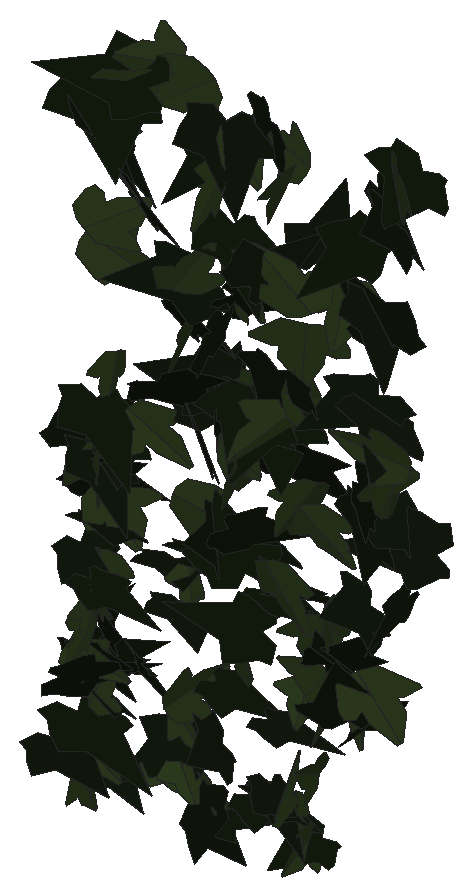
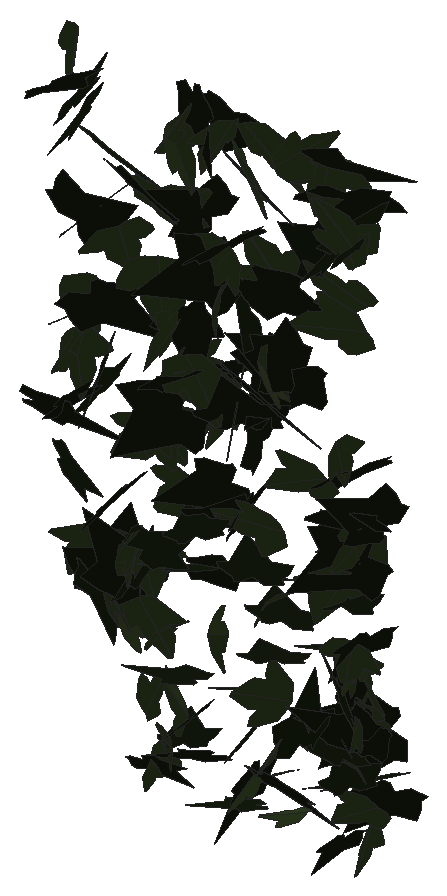
# SketchUp Ruby script. Lengths in inches.
U = 1.inch
M = Sketchup.active_model
def pt(a) = Geom::Point3d.new(a.map { |v| v * U })
def face(e, loops, mat)
  f = e.add_face(loops[0].map { |a| pt(a) })
  loops[1..].each { |l| e.add_face(l.map { |a| pt(a) }).erase! }
  f.material = f.back_material = mat if mat
  f
end
# faces: each face lists its corners as indices into pts; further lists are holes
def faces(e, pts, list, mat = nil) = list.each { |f| face(e, (f[0].is_a?(Array) ? f : [f]).map { |l| l.map { |i| pts[i] } }, mat) }
# xy, xz, yz: faces in a plane at the given z, y or x. An outline is a flat list of corners, or four numbers for a rectangle; further outlines are holes
def ring(l) = l.size == 4 ? [[l[0], l[1]], [l[2], l[1]], [l[2], l[3]], [l[0], l[3]]] : l.each_slice(2).to_a
def flat(e, list, mat, &to3) = list.each { |f| face(e, (f[0].is_a?(Array) ? f : [f]).map { |l| ring(l).map { |u, v| to3.(u, v) } }, mat) }
def xy(e, z, list, mat = nil) = flat(e, list, mat) { |x, y| [x, y, z] }
def xz(e, y, list, mat = nil) = flat(e, list, mat) { |x, z| [x, y, z] }
def yz(e, x, list, mat = nil) = flat(e, list, mat) { |y, z| [x, y, z] }
def lines(e, pts, list) = list.each { |a, b| e.add_line(pt(pts[a]), pt(pts[b])) }
# prism: a flat outline (further loops are holes) pulled along v
def prism(e, loops, v, mat = nil)
  f = face(e, loops, mat); d = Geom::Vector3d.new(v.map { |x| x * U })
  f.pushpull(f.normal.samedirection?(d) ? d.length : -d.length)
end
def box(e, o, s, mat = nil) = prism(e, [[o, [o[0] + s[0], o[1], o[2]], [o[0] + s[0], o[1] + s[1], o[2]], [o[0], o[1] + s[1], o[2]]]], [0, 0, s[2]], mat)
def at(x, y, z, deg = 0) = Geom::Transformation.translation(pt([x, y, z])) * Geom::Transformation.rotation(ORIGIN, Z_AXIS, deg.degrees)
def axes(o, x, y, z) = Geom::Transformation.new([*x, 0, *y, 0, *z, 0, *pt(o).to_a, 1])
def part(name) = M.definitions.add(name)
# library, detail: a bought-in or finely detailed component or shape, given as its bounding box
def library(name, o, s) = part(name).tap { |d| box(d.entities, o, s) }
def detail(e, o, s) = box(e.add_group.entities, o, s)
def put(e, d, t, mat = nil) = e.add_instance(d, t).tap { |i| i.material = mat if mat }
def group(e, t, mat = nil) = e.add_group.tap { |g| g.transformation = t; g.material = mat if mat }.entities
root = M.entities
M.materials.add("1026 AP 7946 SUNNY SIDE UP").color = [254, 231, 186]
M.materials.add("efeu1").color = [18, 25, 13]
M.materials.add("efeu2").color = [43, 57, 29]
c1 = part("ivyleaf_9")
p = [[1.54,2.16,1.25],[1.36,2.04,1.19],[-0.21,0.99,0.68],[-0.71,1.11,0.82],[-0.85,0.86,0.67],[-0.8,0.17,0.21],
  [-0.9,-0.01,0.1],[-0.67,-0.16,-0.02],[-0.08,-0.08,-0.05],[-0.03,-0.6,-0.4],[0.65,-0.88,-0.66],[0.83,-0.6,-0.49],
  [1.29,-0.42,-0.43],[1.8125,-0.07,-0.26],[1.21,0.44,0.15]]
faces(c1.entities,p,[[0,1,2,3,4,5,6,7,8,9,10,11,12,13,14]],"efeu1")
c2 = part("ivyleaf_10")
p = [[0,0.5,-0.03],[-0.0625,2.02,-0.43],[-0.19,2.01,-0.46],[-0.54,1.05,-0.29],[-0.52,0.625,-0.18],[-0.83,0.76,-0.28],
  [-1.16,0.64,-0.33],[-1.15,0.33,-0.24],[-0.77,-0.39,0.02],[-0.3,-0.51,0.16],[0.04,-0.48,0.23],[-0.02,2.01,-0.4375],
  [-0.06,2.01,-0.43],[0.04,-0.49,0.23],[0.67,-0.49,0.14],[1.38,0.36,-0.2],[1.375,0.51,-0.24],[0.81,0.65,-0.19],
  [0.62,0.59,-0.15],[0.6,1.09,-0.28],[0.5,1.23,-0.31]]
faces(c2.entities,p,[[0,1,2,3,4,5,6,7,8,9,10],[11,12,0,13,14,15,16,17,18,19,20]],"efeu2")
put(root,c1,axes([140.07,210.01,274.99],[0.40178,0.27327,0.06244],[0.08476,0.03035,-0.38477],[-0.43136,0.26049,-0.01745]),"1026 AP 7946 SUNNY SIDE UP")
put(root,c1,axes([138.16,210.15,268.72],[-0.04545,-0.15248,-0.27536],[0.07021,0.26267,-0.15833],[0.47756,-0.05313,-0.00293]),"1026 AP 7946 SUNNY SIDE UP")
put(root,c2,axes([140.75,210.3125,278.22],[0.38972,-0.31524,0.01139],[-0.01605,-0.02434,-0.41257],[0.49583,0.24698,-0.0223]),"1026 AP 7946 SUNNY SIDE UP")
put(root,c2,axes([142.29,210.24,276.97],[0.41137,0.1162,0.24439],[-0.36093,-0.06335,0.2932],[0.20366,-0.34698,0.02599]),"1026 AP 7946 SUNNY SIDE UP")
put(root,c1,axes([143.24,210.53,273.7],[-0.01,-0.29094,0.24842],[-0.01209,-0.24268,-0.30121],[0.59572,-0.00981,-0.00194]),"1026 AP 7946 SUNNY SIDE UP")
put(root,c2,axes([141.83,210.3,272.5],[-0.43233,0.13643,-0.20668],[0.24343,-0.13631,-0.31365],[-0.29504,-0.31238,0.04407]),"1026 AP 7946 SUNNY SIDE UP")
put(root,c2,axes([140.28,210.22,276.53],[-0.24834,-0.27881,0.12117],[0.07338,0.11045,0.33049],[-0.47111,0.16418,-0.01239]),"1026 AP 7946 SUNNY SIDE UP")
put(root,c2,axes([141.3125,210.05,274.09],[0.037,-0.24145,-0.32858],[0.04753,0.31829,-0.24513],[0.62549,-0.0099,0.03806]),"1026 AP 7946 SUNNY SIDE UP")
put(root,c2,axes([141.61,210.55,274.69],[-0.09782,-0.18167,0.35137],[-0.02071,-0.34529,-0.19339],[0.60871,-0.04095,0.04988]),"1026 AP 7946 SUNNY SIDE UP")
put(root,c2,axes([138.46,210.39,270.53],[0.3277,-0.2593,0.03455],[0.00983,-0.03981,-0.34233],[0.4113,0.20754,-0.01935]),"1026 AP 7946 SUNNY SIDE UP")
put(root,c1,axes([140.87,210.43,279.06],[-0.41385,-0.1169,-0.29365],[0.4378,0.06819,-0.29395],[0.20511,-0.38143,0.03493]),"1026 AP 7946 SUNNY SIDE UP")
put(root,c2,axes([143.83,210.3,274.96],[-0.05411,-0.01018,-0.34825],[-0.52122,0.06812,0.03305],[0.10502,0.33284,-0.01538]),"1026 AP 7946 SUNNY SIDE UP")
put(root,c1,axes([138.63,210.45,273.98],[0.01166,-0.37789,-0.0741],[0.05587,0.07017,-0.38717],[0.60166,0.00081,0.03739]),"1026 AP 7946 SUNNY SIDE UP")
put(root,c1,axes([141.39,210.44,271.42],[-0.22535,-0.18226,-0.2308],[-0.25475,-0.15493,0.2368],[-0.37442,0.2151,-0.0222]),"1026 AP 7946 SUNNY SIDE UP")
put(root,c1,axes([142.98,210.42,270.63],[0.44825,0.10129,0.24697],[-0.37465,-0.03936,0.30952],[0.16255,-0.37002,0.03233]),"1026 AP 7946 SUNNY SIDE UP")
put(root,c1,axes([141.57,210.12,277.01],[-0.0766,0.01171,0.37077],[0.48224,0.19153,0.03747],[-0.2965,0.30849,-0.03484]),"1026 AP 7946 SUNNY SIDE UP")
put(root,c1,axes([139.14,210.53,277.39],[0.19991,-0.19654,0.25854],[0.17933,-0.22554,-0.24173],[0.46953,0.16982,-0.01775]),"1026 AP 7946 SUNNY SIDE UP")
put(root,c1,axes([140.68,210.6,272.46],[-0.0974,-0.05315,0.33824],[-0.19734,-0.30588,-0.07712],[0.48483,-0.13518,0.03656]),"1026 AP 7946 SUNNY SIDE UP")
put(root,c1,axes([141.27,210.58,274.76],[-0.29544,-0.3241,0.03258],[-0.00135,-0.03813,-0.3857],[0.51232,-0.187,0.01777]),"1026 AP 7946 SUNNY SIDE UP")
put(root,c1,axes([140.32,210.47,276.49],[-0.07315,-0.04963,-0.36518],[-0.41399,-0.237,0.06845],[-0.38063,0.26731,-0.00427]),"1026 AP 7946 SUNNY SIDE UP")
put(root,c2,axes([141.13,210.18,274.3125],[-0.03447,0.29802,0.24234],[-0.05526,0.23132,-0.30614],[-0.59278,-0.03889,0.01445]),"1026 AP 7946 SUNNY SIDE UP")
put(root,c1,axes([143.59,210.66,278.38],[0.22834,-0.24967,-0.20641],[0.18571,-0.16104,0.29606],[-0.46635,-0.18637,0.01684]),"1026 AP 7946 SUNNY SIDE UP")
put(root,c2,axes([138.53,210.55,272.97],[0.127,-0.16358,0.22614],[0.2457,-0.16152,-0.1834],[0.35487,0.17038,0.04605]),"1026 AP 7946 SUNNY SIDE UP")
put(root,c1,axes([138.28,210.15,269.75],[0.0981,0.25276,-0.26663],[0.07124,0.25657,0.2694],[0.56599,-0.07611,0.0123]),"1026 AP 7946 SUNNY SIDE UP")
put(root,c1,axes([140.16,210.66,274.05],[0.2445,-0.12889,-0.34122],[0.47304,-0.14328,0.20255],[-0.29555,-0.33596,0.04191]),"1026 AP 7946 SUNNY SIDE UP")
put(root,c1,axes([138.3125,210.47,269.02],[0.16537,-0.34706,-0.11032],[0.20846,0.13867,-0.33421],[0.53073,0.05367,0.16565]),"1026 AP 7946 SUNNY SIDE UP")
put(root,c1,axes([138.54,210.57,273.08],[0.05294,-0.35255,0.00123],[0.05448,0.00011,-0.36311],[0.5517,0.03382,0.03574]),"1026 AP 7946 SUNNY SIDE UP")
put(root,c1,axes([140.82,210.11,275.68],[-0.00325,0.2124,0.36129],[0.018,0.34939,-0.21664],[-0.64282,0.00871,-0.00789]),"1026 AP 7946 SUNNY SIDE UP")
put(root,c2,axes([138.46,210.52,270.78],[-0.02236,-0.282,0.06478],[0.11002,-0.06599,-0.28182],[0.44135,0.00217,0.07353]),"1026 AP 7946 SUNNY SIDE UP")
put(root,c2,axes([141.89,210.34,268.85],[0.31294,-0.29045,0.20104],[-0.14118,0.17656,0.36302],[-0.5333,-0.21718,0.02187]),"1026 AP 7946 SUNNY SIDE UP")
put(root,c1,axes([138.47,210.66,270.48],[0.03791,-0.07198,0.30482],[0.12491,-0.28547,-0.07978],[0.46289,0.08293,-0.00344]),"1026 AP 7946 SUNNY SIDE UP")
put(root,c2,axes([143.31,210.39,271.25],[0.31372,0.29588,0.15478],[0.1569,0.11165,-0.36648],[-0.4964,0.22229,-0.01801]),"1026 AP 7946 SUNNY SIDE UP")
put(root,c2,axes([138.33,210.45,268.09],[0.04349,-0.27871,-0.09833],[0.14188,0.09778,-0.27112],[0.44013,-0.00398,0.09711]),"1026 AP 7946 SUNNY SIDE UP")
put(root,c1,axes([140.78,210.35,274.65],[0.20945,-0.12552,-0.34184],[-0.44154,0.17807,-0.18488],[0.3392,0.3093,-0.02958]),"1026 AP 7946 SUNNY SIDE UP")
put(root,c2,axes([138.64,210.43,276.8],[0.35877,-0.01709,-0.25478],[0.38807,0.04585,0.23167],[0.03499,-0.33327,0.04294]),"1026 AP 7946 SUNNY SIDE UP")
put(root,c1,axes([138.52,210.5,271.16],[0.20671,-0.23217,-0.07785],[0.18431,0.13418,-0.21764],[0.33606,0.06922,0.16725]),"1026 AP 7946 SUNNY SIDE UP")
put(root,c1,axes([141.15,210.43,272.29],[-0.48396,-0.12451,0.09323],[0.11331,0.064,0.3409],[-0.21461,0.31457,-0.03025]),"1026 AP 7946 SUNNY SIDE UP")
put(root,c1,axes([143.19,210.4,274.3125],[0.28747,-0.18472,-0.30659],[-0.37351,0.17972,-0.26514],[0.40285,0.29844,-0.02705]),"1026 AP 7946 SUNNY SIDE UP")
put(root,c1,axes([141.72,210.45,275.54],[0.35366,0.04247,-0.27847],[-0.40556,-0.08484,-0.23511],[-0.14476,0.34144,-0.02163]),"1026 AP 7946 SUNNY SIDE UP")
put(root,c1,axes([141.52,210.59,268.97],[0.13736,-0.29429,-0.06582],[-0.03901,0.05753,-0.31583],[0.47136,0.09052,-0.00695]),"1026 AP 7946 SUNNY SIDE UP")
put(root,c1,axes([143.08,210.6875,277.91],[-0.57651,0.04642,-0.1139],[0.14614,-0.11597,-0.36748],[-0.11974,-0.36505,0.09988]),"1026 AP 7946 SUNNY SIDE UP")
put(root,c2,axes([143.79,210.46,279.29],[-0.32504,0.2957,0.07107],[-0.12294,0.02673,-0.36823],[-0.46074,-0.21575,0.04813]),"1026 AP 7946 SUNNY SIDE UP")
put(root,c2,axes([138.31,210.43,269.98],[0.15763,0.07754,0.25521],[0.29081,0.16434,-0.12936],[-0.28547,0.21022,0.00914]),"1026 AP 7946 SUNNY SIDE UP")
put(root,c2,axes([139.93,210.67,268.61],[-0.17579,-0.21006,0.0807],[0.27865,-0.13707,-0.11714],[0.21699,0.00585,0.21581]),"1026 AP 7946 SUNNY SIDE UP")
put(root,c1,axes([140.45,210.4,268.37],[0.19173,-0.19281,-0.33756],[-0.2876,0.2706,-0.23336],[0.52238,0.21975,-0.00459]),"1026 AP 7946 SUNNY SIDE UP")
put(root,c1,axes([141.5,210.75,268.67],[-0.1951,-0.16948,0.14734],[0.15714,-0.18978,-0.14253],[0.31238,-0.01038,0.16372]),"1026 AP 7946 SUNNY SIDE UP")
put(root,c2,axes([138.3,210.51,268.57],[0.26494,0.08808,0.2064],[0.2925,0.07437,-0.1949],[-0.17993,0.25059,-0.01293]),"1026 AP 7946 SUNNY SIDE UP")
put(root,c2,axes([142.05,210.71,273.69],[-0.11028,-0.30817,0.17232],[-0.04834,-0.16631,-0.3265],[0.55054,-0.07633,0.00585]),"1026 AP 7946 SUNNY SIDE UP")
put(root,c1,axes([138.59,210.76,271.95],[-0.20299,-0.21447,0.11334],[0.27957,-0.16973,-0.12554],[0.25721,0.01522,0.2259]),"1026 AP 7946 SUNNY SIDE UP")
put(root,c2,axes([142.21,210.58,273.41],[-0.43522,0.02313,-0.20772],[0.30891,-0.05592,-0.28458],[-0.0809,-0.33792,0.03083]),"1026 AP 7946 SUNNY SIDE UP")
put(root,c1,axes([143.15,210.81,276.82],[0.01646,-0.36633,0.09706],[-0.01372,-0.09654,-0.37793],[0.59543,0.0079,-0.01139]),"1026 AP 7946 SUNNY SIDE UP")
put(root,c1,axes([138.56,210.71,278.67],[-0.30132,-0.30811,-0.16871],[0.16401,0.12563,-0.37247],[0.52222,-0.21723,0.01963]),"1026 AP 7946 SUNNY SIDE UP")
put(root,c2,axes([138.6,210.55,276.37],[0.2007,0.06087,0.36455],[0.53485,0.09863,-0.14344],[-0.17914,0.36268,-0.01984]),"1026 AP 7946 SUNNY SIDE UP")
put(root,c1,axes([141.01,210.36,272.9],[0.04168,0.11869,-0.31148],[0.02689,0.3031,0.12562],[0.51101,-0.02563,0.0188]),"1026 AP 7946 SUNNY SIDE UP")
put(root,c2,axes([138.46,210.53,270.98],[0.27482,-0.20285,-0.07137],[0.14175,0.14957,-0.21969],[0.30515,0.11321,0.16632]),"1026 AP 7946 SUNNY SIDE UP")
put(root,c1,axes([138.2,210.39,273.24],[-0.05434,0.00938,0.35574],[0.45794,0.18732,0.02589],[-0.29195,0.29208,-0.02561]),"1026 AP 7946 SUNNY SIDE UP")
put(root,c2,axes([142.06,210.65,276.15],[-0.52196,-0.21381,0.02804],[0.01445,-0.06615,-0.40236],[0.33885,-0.32653,0.06035]),"1026 AP 7946 SUNNY SIDE UP")
put(root,c2,axes([140.875,210.66,276.83],[-0.43381,0.16439,-0.16652],[0.1757,-0.12678,-0.32816],[-0.31826,-0.29406,0.04581]),"1026 AP 7946 SUNNY SIDE UP")
put(root,c1,axes([143.28,210.89,275.18],[-0.17956,-0.31962,0.14241],[0.02507,-0.15199,-0.34483],[0.54814,-0.09775,0.06242]),"1026 AP 7946 SUNNY SIDE UP")
put(root,c1,axes([139.19,210.75,278.95],[-0.35447,0.03525,0.30938],[-0.47461,-0.04393,-0.22852],[0.0224,-0.37277,0.05395]),"1026 AP 7946 SUNNY SIDE UP")
put(root,c2,axes([141.7,210.7,278.48],[0.06748,-0.39156,0.03011],[0.00006,-0.03163,-0.40597],[0.61768,0.04278,-0.00325]),"1026 AP 7946 SUNNY SIDE UP")
put(root,c2,axes([138.375,210.49,273.01],[-0.17651,-0.19276,-0.24382],[0.20666,0.19578,-0.2284],[0.43171,-0.17253,0.00965]),"1026 AP 7946 SUNNY SIDE UP")
put(root,c2,axes([143.54,210.65,274.45],[-0.0979,-0.37448,-0.03451],[0.03495,0.02808,-0.39051],[0.58986,-0.06382,0.01741]),"1026 AP 7946 SUNNY SIDE UP")
put(root,c1,axes([138.59,210.74,273.37],[-0.26335,-0.22435,-0.11724],[0.12346,0.08166,-0.28764],[0.37485,-0.18451,0.01237]),"1026 AP 7946 SUNNY SIDE UP")
put(root,c1,axes([140.45,210.75,278.4],[-0.48775,0.0933,-0.12876],[0.16791,-0.07734,-0.33155],[-0.17967,-0.32557,0.03969]),"1026 AP 7946 SUNNY SIDE UP")
put(root,c2,axes([141.97,210.86,268.2],[0.03165,0.14265,-0.29089],[-0.1135,-0.27423,-0.14921],[-0.48548,0.07341,0.01592]),"1026 AP 7946 SUNNY SIDE UP")
put(root,c1,axes([143.67,210.8,272.5625],[-0.34787,0.07548,-0.21945],[0.25828,-0.15188,-0.23161],[-0.245,-0.26728,0.06744]),"1026 AP 7946 SUNNY SIDE UP")
put(root,c1,axes([141.45,210.84,274.7],[-0.21306,-0.34949,-0.05577],[0.07662,0.03684,-0.38455],[0.55032,-0.14044,0.03195]),"1026 AP 7946 SUNNY SIDE UP")
put(root,c1,axes([140.34,210.95,269.08],[-0.12759,-0.14037,0.30522],[-0.11184,-0.29124,-0.16349],[0.50439,-0.10009,0.04096]),"1026 AP 7946 SUNNY SIDE UP")
put(root,c1,axes([138.25,210.59,269.98],[0.4834,0.02841,-0.019],[-0.02467,-0.03149,-0.31675],[-0.04736,0.30637,-0.02896]),"1026 AP 7946 SUNNY SIDE UP")
put(root,c1,axes([143.25,210.5,270.6],[-0.05523,0.30228,0.08269],[-0.01645,0.07786,-0.31305],[-0.49082,-0.03663,0.00119]),"1026 AP 7946 SUNNY SIDE UP")
put(root,c2,axes([140.9,210.58,278.86],[0.06556,0.36801,0.09584],[0.02895,0.08942,-0.38093],[-0.59536,0.04487,-0.00797]),"1026 AP 7946 SUNNY SIDE UP")
put(root,c1,axes([143.09,210.85,275.47],[0.03831,0.01643,-0.3598],[-0.17092,-0.33249,-0.02587],[-0.52268,0.10993,-0.01791]),"1026 AP 7946 SUNNY SIDE UP")
put(root,c2,axes([138.61,210.8,274.46],[-0.02402,-0.29302,0.0967],[0.11831,-0.0963,-0.29247],[0.46995,0.00927,0.07857]),"1026 AP 7946 SUNNY SIDE UP")
put(root,c1,axes([138.14,210.85,278.26],[0.30597,-0.38066,0.0551],[0.01725,-0.05685,-0.44045],[0.60467,0.19424,-0.01532]),"1026 AP 7946 SUNNY SIDE UP")
put(root,c2,axes([142.38,210.94,270.45],[0.12293,-0.18044,0.29105],[0.12258,-0.27344,-0.20301],[0.51406,0.10835,-0.02119]),"1026 AP 7946 SUNNY SIDE UP")
put(root,c1,axes([142.86,210.99,272.08],[0.14583,-0.2465,-0.23525],[0.15822,-0.20413,0.26957],[-0.50255,-0.1358,0.01661]),"1026 AP 7946 SUNNY SIDE UP")
put(root,c1,axes([140.64,210.87,277.2],[0.00257,-0.39197,-0.04097],[0.03434,0.03758,-0.40296],[0.61821,-0.00046,0.02256]),"1026 AP 7946 SUNNY SIDE UP")
put(root,c2,axes([142.02,210.94,269.2],[-0.02724,-0.12531,-0.28375],[-0.06806,-0.2713,0.12871],[-0.46988,0.04656,-0.00219]),"1026 AP 7946 SUNNY SIDE UP")
put(root,c1,axes([138.17,210.6875,271.5],[0.08916,-0.25562,-0.20869],[-0.06172,0.19729,-0.26856],[0.5077,0.06888,0.004]),"1026 AP 7946 SUNNY SIDE UP")
put(root,c2,axes([143.51,210.48,274.58],[0.03623,-0.18683,-0.36145],[0.15501,0.34209,-0.17953],[0.60399,-0.07659,0.06776]),"1026 AP 7946 SUNNY SIDE UP")
put(root,c2,axes([139.86,210.87,271.52],[-0.09761,-0.2139,0.15219],[0.2295,-0.15538,-0.16813],[0.33956,0.04353,0.15738]),"1026 AP 7946 SUNNY SIDE UP")
put(root,c2,axes([139.84,210.92,275.43],[0.20786,-0.28218,0.2124],[0.10585,-0.19749,-0.32158],[0.54075,0.14712,-0.0187]),"1026 AP 7946 SUNNY SIDE UP")
put(root,c2,axes([138.91,210.72,278.97],[-0.41006,-0.22608,-0.04542],[0.07593,0.00948,-0.35462],[0.35374,-0.26411,0.02347]),"1026 AP 7946 SUNNY SIDE UP")
put(root,c2,axes([139.16,210.6875,273.78],[0.27229,0.09594,0.27801],[0.40579,0.08304,-0.20094],[-0.19345,0.30923,-0.03018]),"1026 AP 7946 SUNNY SIDE UP")
put(root,c2,axes([138.37,210.72,269.22],[0.35705,-0.16538,-0.03712],[0.06509,-0.00259,0.28849],[-0.25775,-0.22976,0.02143]),"1026 AP 7946 SUNNY SIDE UP")
put(root,c1,axes([141.4375,210.63,279.22],[0.21836,-0.06099,-0.34277],[-0.52388,0.0354,-0.14989],[0.08888,0.35848,-0.04134]),"1026 AP 7946 SUNNY SIDE UP")
put(root,c2,axes([141.81,210.92,270.4],[-0.2036,-0.13891,0.18807],[0.16415,-0.22297,-0.09939],[0.3223,0.02581,0.16943]),"1026 AP 7946 SUNNY SIDE UP")
put(root,c1,axes([140.09,210.9375,271.98],[-0.18903,-0.22108,0.09829],[0.29968,-0.15324,-0.11776],[0.23268,0.01775,0.23152]),"1026 AP 7946 SUNNY SIDE UP")
put(root,c1,axes([140.52,210.66,274.86],[-0.3679,0.24322,0.19646],[-0.25998,0.10155,-0.34431],[-0.40901,-0.28332,0.04215]),"1026 AP 7946 SUNNY SIDE UP")
put(root,c1,axes([138.3,210.95,269.17],[-0.10957,-0.1902,0.18902],[0.20431,-0.19084,-0.15319],[0.36321,0.04997,0.14319]),"1026 AP 7946 SUNNY SIDE UP")
put(root,c2,axes([139.93,210.8125,272.75],[-0.12287,-0.0351,-0.33532],[0.49036,-0.10917,-0.06568],[-0.15565,-0.31624,0.0578]),"1026 AP 7946 SUNNY SIDE UP")
put(root,c1,axes([140.99,210.51,276.45],[0.35664,0.17904,0.26579],[0.36044,0.12131,-0.29479],[-0.33558,0.32057,-0.03415]),"1026 AP 7946 SUNNY SIDE UP")
put(root,c1,axes([143.55,211.04,273.59],[-0.17889,-0.15607,0.26062],[-0.18838,-0.22485,-0.19904],[0.42904,-0.1638,0.02127]),"1026 AP 7946 SUNNY SIDE UP")
put(root,c2,axes([139.99,210.53,269.8],[0.01524,-0.17343,0.36752],[-0.02011,0.35752,0.18101],[-0.62479,-0.01574,0.00314]),"1026 AP 7946 SUNNY SIDE UP")
put(root,c1,axes([139.15,211.03,269.63],[0.40108,-0.26089,-0.11311],[0.14973,-0.05798,0.37456],[-0.41818,-0.27098,0.02563]),"1026 AP 7946 SUNNY SIDE UP")
put(root,c1,axes([139.43,210.95,275.62],[0.26826,-0.18675,0.27874],[0.2608,-0.21568,-0.26134],[0.44792,0.23742,-0.01477]),"1026 AP 7946 SUNNY SIDE UP")
put(root,c1,axes([138.34,210.58,272.72],[0.41857,0.18895,0.1697],[0.23955,0.06691,-0.33448],[-0.31163,0.30523,-0.02918]),"1026 AP 7946 SUNNY SIDE UP")
put(root,c1,axes([144.07,210.85,273.38],[-0.44546,0.09606,0.21021],[-0.32612,0.01553,-0.3049],[-0.13733,-0.34847,0.04217]),"1026 AP 7946 SUNNY SIDE UP")
put(root,c2,axes([141.92,210.54,275.22],[-0.05729,0.15658,0.3409],[-0.15052,0.31597,-0.16349],[-0.5543,-0.10199,0.00916]),"1026 AP 7946 SUNNY SIDE UP")
put(root,c1,axes([143.47,210.71,276.54],[0.08762,-0.03845,0.39183],[-0.38968,0.28932,0.06919],[-0.45814,-0.25344,0.01609]),"1026 AP 7946 SUNNY SIDE UP")
put(root,c2,axes([138.37,210.79,270.02],[-0.30252,0.17151,-0.02669],[0.00517,-0.03652,-0.26449],[-0.27293,-0.1908,0.02458]),"1026 AP 7946 SUNNY SIDE UP")
put(root,c1,axes([142.0625,210.93,268.23],[-0.36622,-0.07208,0.03681],[-0.04617,-0.02707,-0.25071],[0.11807,-0.23413,0.01613]),"1026 AP 7946 SUNNY SIDE UP")
put(root,c2,axes([142.1875,210.87,271.625],[-0.26401,-0.30496,0.0491],[-0.01696,-0.05039,-0.35861],[0.48547,-0.1676,0.01417]),"1026 AP 7946 SUNNY SIDE UP")
put(root,c2,axes([141.68,210.92,268.66],[-0.20055,0.13376,-0.17134],[0.07347,-0.1724,-0.17995],[-0.32842,-0.12025,0.06437]),"1026 AP 7946 SUNNY SIDE UP")
put(root,c1,axes([141.06,210.76,268.61],[0.19638,-0.15416,-0.16726],[0.16587,0.20383,-0.11522],[0.30939,-0.01142,0.16794]),"1026 AP 7946 SUNNY SIDE UP")
put(root,c2,axes([142.6,210.98,270.64],[0.31765,-0.1394,0.2485],[0.31384,-0.13687,-0.25365],[0.30718,0.28398,0.00218]),"1026 AP 7946 SUNNY SIDE UP")
put(root,c1,axes([140.49,210.71,274.28],[-0.4157,-0.05281,0.24456],[0.3614,0.06171,0.27784],[-0.12641,0.35012,-0.00992]),"1026 AP 7946 SUNNY SIDE UP")
put(root,c2,axes([141.32,210.83,274.87],[-0.51057,0.00603,0.20003],[-0.30399,-0.04633,-0.33192],[0.02931,-0.37547,0.04194]),"1026 AP 7946 SUNNY SIDE UP")
put(root,c1,axes([138.32,210.74,269.82],[0.04618,0.01008,0.29306],[0.4448,0.03028,-0.03102],[-0.04901,0.28432,-0.0054]),"1026 AP 7946 SUNNY SIDE UP")
put(root,c1,axes([142.32,210.82,271.09],[0.39835,0.23541,0.02904],[-0.05831,0.00057,0.3553],[0.36796,-0.25476,0.02487]),"1026 AP 7946 SUNNY SIDE UP")
put(root,c2,axes([138.36,210.87,271.31],[-0.41568,-0.01215,-0.02659],[0.04363,-0.05618,-0.26653],[0.01001,-0.2596,0.05733]),"1026 AP 7946 SUNNY SIDE UP")
put(root,c1,axes([142.2,211.1,271.18],[0.28931,-0.24284,-0.15451],[0.16764,-0.10529,0.31263],[-0.41509,-0.21178,0.01857]),"1026 AP 7946 SUNNY SIDE UP")
put(root,c2,axes([141.66,210.99,278.55],[-0.14072,0.27315,0.18068],[0.01975,-0.17729,0.29261],[0.50872,0.08244,0.03862]),"1026 AP 7946 SUNNY SIDE UP")
put(root,c1,axes([141.31,210.85,269.82],[0.26103,-0.20166,-0.02699],[0.22877,0.14053,-0.17136],[0.22308,0.09185,0.20732]),"1026 AP 7946 SUNNY SIDE UP")
put(root,c1,axes([138.56,210.9,277.86],[0.277,-0.24363,-0.08706],[-0.09384,0.05932,-0.30908],[0.39373,0.18554,-0.01242]),"1026 AP 7946 SUNNY SIDE UP")
put(root,c1,axes([138.38,210.91,270.35],[-0.02221,0.20846,0.20982],[0.02111,-0.20204,0.21406],[0.45648,0.01949,0.00031]),"1026 AP 7946 SUNNY SIDE UP")
put(root,c1,axes([140.25,210.74,268.06],[0.36788,-0.06561,-0.0619],[0.0499,0.21917,-0.1187],[0.13026,0.10133,0.22029]),"1026 AP 7946 SUNNY SIDE UP")
put(root,c2,axes([138.24,210.97,277.9],[-0.30657,0.0951,0.24744],[0.35428,-0.08321,0.22238],[0.19708,0.29752,-0.01484]),"1026 AP 7946 SUNNY SIDE UP")
put(root,c1,axes([141.02,211.09,272.39],[-0.12637,-0.22813,0.14395],[0.20168,-0.16199,-0.1956],[0.37038,0.01037,0.15562]),"1026 AP 7946 SUNNY SIDE UP")
put(root,c2,axes([142.13,210.93,270.71],[-0.48794,-0.01012,0.16586],[-0.23578,-0.11093,-0.30547],[0.09377,-0.33156,0.09498]),"1026 AP 7946 SUNNY SIDE UP")
put(root,c2,axes([140.22,210.79,268.46],[0.21874,-0.18868,-0.09976],[0.1666,0.16132,-0.16794],[0.28799,0.04999,0.17292]),"1026 AP 7946 SUNNY SIDE UP")
put(root,c2,axes([138.57,210.78,272.35],[0.29366,0.30021,0.14654],[0.09023,0.1296,-0.36299],[-0.51336,0.19451,0.02003]),"1026 AP 7946 SUNNY SIDE UP")
put(root,c1,axes([139.4375,211.1,271.55],[-0.18673,-0.24447,0.03972],[0.31757,-0.12121,-0.14634],[0.22553,-0.03174,0.23895]),"1026 AP 7946 SUNNY SIDE UP")
put(root,c1,axes([141.61,210.74,274.07],[0.53269,0.14406,0.05521],[0.09925,-0.01426,-0.37736],[-0.21988,0.34256,-0.03657]),"1026 AP 7946 SUNNY SIDE UP")
put(root,c2,axes([139.25,211.15,279.16],[0.01483,0.1669,0.35432],[-0.04139,-0.34199,0.17019],[0.59835,-0.02779,0.00299]),"1026 AP 7946 SUNNY SIDE UP")
put(root,c2,axes([139.25,210.94,268.34],[0.01026,-0.24941,0.01188],[0.37629,0.00254,-0.07386],[0.11236,0.01428,0.24627]),"1026 AP 7946 SUNNY SIDE UP")
put(root,c2,axes([139.65,210.92,269.28],[0.04824,-0.25671,-0.03594],[0.22537,0.04488,-0.21925],[0.33897,0.0067,0.15088]),"1026 AP 7946 SUNNY SIDE UP")
put(root,c1,axes([138.45,210.9,268.2],[0.08387,-0.20116,-0.1673],[-0.05513,0.15748,-0.21341],[0.40162,0.06362,0.00564]),"1026 AP 7946 SUNNY SIDE UP")
put(root,c2,axes([140.01,210.91,279.21],[0.41355,-0.16123,-0.24006],[-0.33422,0.09611,-0.31634],[0.29287,0.33735,-0.02202]),"1026 AP 7946 SUNNY SIDE UP")
put(root,c1,axes([138.4,211.02,269.62],[0.03946,-0.24915,0.05391],[0.39389,0.01414,-0.0529],[0.074,0.05761,0.25281]),"1026 AP 7946 SUNNY SIDE UP")
put(root,c2,axes([142.49,210.99,276.79],[0.28444,0.31857,-0.12227],[-0.10135,-0.10195,-0.37796],[-0.52588,0.19196,0.00671]),"1026 AP 7946 SUNNY SIDE UP")
put(root,c1,axes([141.91,211.14,271.85],[-0.41349,-0.04492,-0.00159],[0.06871,-0.25383,-0.07307],[0.01646,-0.06871,0.26494]),"1026 AP 7946 SUNNY SIDE UP")
put(root,c1,axes([142.25,210.75,277.4],[-0.44999,0.22773,0.02502],[0.04744,0.00103,0.37624],[0.35676,0.2871,-0.01847]),"1026 AP 7946 SUNNY SIDE UP")
put(root,c1,axes([139.57,211.12,270.86],[-0.12967,-0.25454,0.02581],[0.25202,-0.07308,-0.2097],[0.31372,-0.04651,0.17913]),"1026 AP 7946 SUNNY SIDE UP")
put(root,c1,axes([139.7,211.07,268.83],[-0.54647,0.03476,-0.01168],[0.00961,-0.05352,-0.35602],[-0.05679,-0.34358,0.05219]),"1026 AP 7946 SUNNY SIDE UP")
put(root,c1,axes([143.125,210.94,278.59],[0.30611,-0.2677,-0.14195],[-0.16037,0.09383,-0.33946],[0.44427,0.21832,-0.02473]),"1026 AP 7946 SUNNY SIDE UP")
put(root,c1,axes([143.57,211.21,278.9375],[-0.25856,-0.2772,0.13872],[-0.06408,-0.13351,-0.33133],[0.48142,-0.16665,0.0304]),"1026 AP 7946 SUNNY SIDE UP")
put(root,c2,axes([140.9375,210.74,270.61],[-0.15639,0.16575,-0.31459],[-0.19716,0.28015,0.19975],[0.51091,0.15884,-0.01921]),"1026 AP 7946 SUNNY SIDE UP")
put(root,c1,axes([140.34,210.93,270.03],[0.22598,-0.18536,-0.12175],[0.17193,0.18198,-0.15739],[0.29884,0.03547,0.18262]),"1026 AP 7946 SUNNY SIDE UP")
put(root,c1,axes([141.13,210.95,271.72],[0.22969,-0.20933,-0.08978],[0.21116,0.16254,-0.17171],[0.28639,0.04804,0.19861]),"1026 AP 7946 SUNNY SIDE UP")
put(root,c2,axes([142.29,210.89,271.75],[-0.10031,0.3408,0.07516],[-0.10573,0.05878,-0.35246],[-0.53707,-0.07522,0.05535]),"1026 AP 7946 SUNNY SIDE UP")
put(root,c2,axes([138.26,210.97,278.08],[-0.405,-0.06439,0.19213],[0.26767,0.08371,0.27193],[-0.15793,0.30701,-0.03183]),"1026 AP 7946 SUNNY SIDE UP")
put(root,c2,axes([140.85,210.8,276.08],[-0.12189,0.26055,-0.22753],[-0.07007,0.21836,0.28089],[0.53401,0.08812,-0.01508]),"1026 AP 7946 SUNNY SIDE UP")
